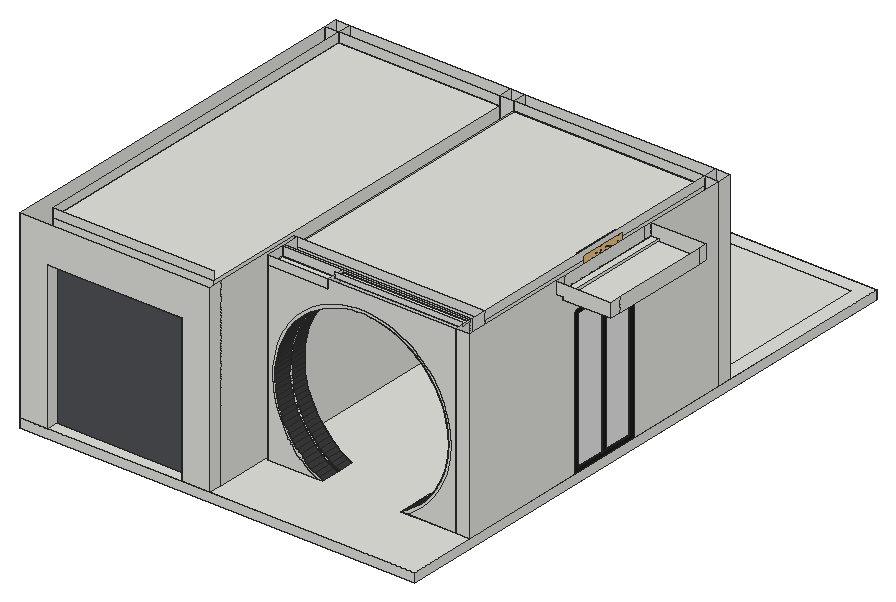
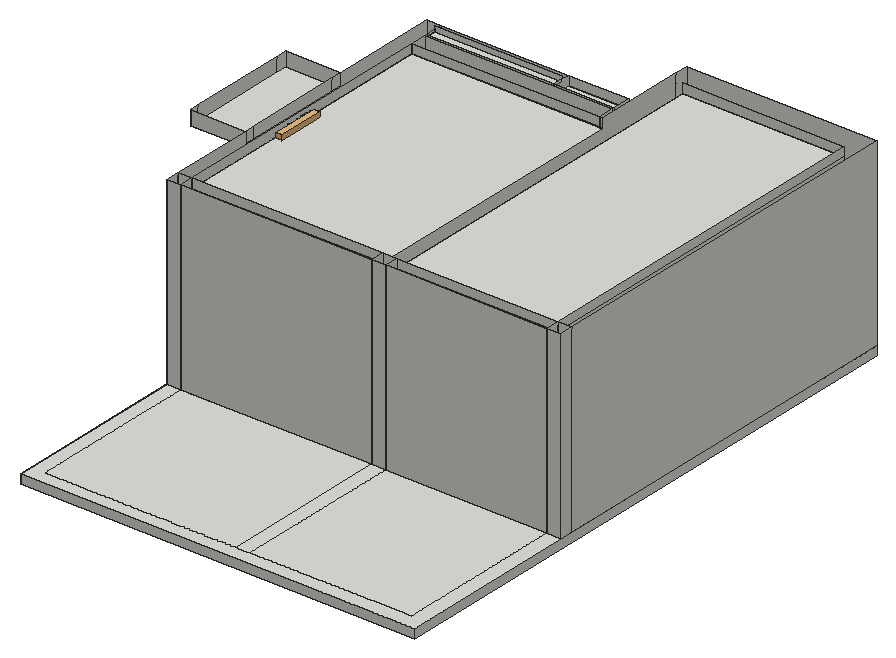
# SketchUp Ruby script. Lengths in inches.
U = 1.inch
M = Sketchup.active_model
def pt(a) = Geom::Point3d.new(a.map { |v| v * U })
def face(e, loops, mat)
  f = e.add_face(loops[0].map { |a| pt(a) })
  loops[1..].each { |l| e.add_face(l.map { |a| pt(a) }).erase! }
  f.material = f.back_material = mat if mat
  f
end
# faces: each face lists its corners as indices into pts; further lists are holes
def faces(e, pts, list, mat = nil) = list.each { |f| face(e, (f[0].is_a?(Array) ? f : [f]).map { |l| l.map { |i| pts[i] } }, mat) }
# xy, xz, yz: faces in a plane at the given z, y or x. An outline is a flat list of corners, or four numbers for a rectangle; further outlines are holes
def ring(l) = l.size == 4 ? [[l[0], l[1]], [l[2], l[1]], [l[2], l[3]], [l[0], l[3]]] : l.each_slice(2).to_a
def flat(e, list, mat, &to3) = list.each { |f| face(e, (f[0].is_a?(Array) ? f : [f]).map { |l| ring(l).map { |u, v| to3.(u, v) } }, mat) }
def xy(e, z, list, mat = nil) = flat(e, list, mat) { |x, y| [x, y, z] }
def xz(e, y, list, mat = nil) = flat(e, list, mat) { |x, z| [x, y, z] }
def yz(e, x, list, mat = nil) = flat(e, list, mat) { |y, z| [x, y, z] }
def lines(e, pts, list) = list.each { |a, b| e.add_line(pt(pts[a]), pt(pts[b])) }
# prism: a flat outline (further loops are holes) pulled along v
def prism(e, loops, v, mat = nil)
  f = face(e, loops, mat); d = Geom::Vector3d.new(v.map { |x| x * U })
  f.pushpull(f.normal.samedirection?(d) ? d.length : -d.length)
end
def box(e, o, s, mat = nil) = prism(e, [[o, [o[0] + s[0], o[1], o[2]], [o[0] + s[0], o[1] + s[1], o[2]], [o[0], o[1] + s[1], o[2]]]], [0, 0, s[2]], mat)
def at(x, y, z, deg = 0) = Geom::Transformation.translation(pt([x, y, z])) * Geom::Transformation.rotation(ORIGIN, Z_AXIS, deg.degrees)
def axes(o, x, y, z) = Geom::Transformation.new([*x, 0, *y, 0, *z, 0, *pt(o).to_a, 1])
def part(name) = M.definitions.add(name)
# library, detail: a bought-in or finely detailed component or shape, given as its bounding box
def library(name, o, s) = part(name).tap { |d| box(d.entities, o, s) }
def detail(e, o, s) = box(e.add_group.entities, o, s)
def put(e, d, t, mat = nil) = e.add_instance(d, t).tap { |i| i.material = mat if mat }
def group(e, t, mat = nil) = e.add_group.tap { |g| g.transformation = t; g.material = mat if mat }.entities
root = M.entities
M.materials.add("[Blinds Roman Hobbled Blue]").color = [81, 82, 87]
M.materials.add("[Color M07]").color = [58, 58, 58]
M.materials.add("[Color M08]").color = [30, 30, 30]
M.materials.add("[Mirror 02]").color = [229, 229, 229]
c1 = library("Curtains 004",[-15.59,-2.26,0],[31.18,4.52,116.91])
xy(root,-6,[[0,37.13,258,415.13]])
xy(root,0,[[0,37.13,18,37.13,18,44.38,106,44.38,106,37.13,124,37.13,124,286.13,115,286.13,115,52.07,9,52.07,9,286.13,0,286.13],[18,37.13,106,44.38],[[124,37.13,258,37.13,258,82.13,213,82.13,213,106.13,249,106.13,249,286.13,124,286.13],[126,82.13,162,106.13]],[9,52.07,115,286.13],[126,82.13,162,94.13],
  [213,82.13,249,94.13],[249,82.13,258,168.32],[126,94.13,162,95.7],[213,94.13,249,95.7],[126,95.7,162,106.13],
  [213,95.7,249,106.13],[249,216.32,258,286.13],[0,286.13,9,295.13],[9,286.13,115,295.13],[115,286.13,124,295.13],
  [124,286.13,249,295.13],[249,286.13,258,295.13],[0,295.13,9,295.13,9,406.13,249,406.13,249,295.13,258,295.13,258,415.13,0,415.13],[9,295.13,115,406.13],[115,295.13,124,406.13],
  [124,295.13,249,406.13]])
xy(root,0,[[254.4375,168.32,258,216.32]],"[Color M08]")
xy(root,2.75,[[256.5625,171.07,258,191.29],[256.5625,193.38,258,213.57]],"[Color M08]")
xy(root,93.25,[[256.5625,171.07,258,191.29],[256.5625,193.38,258,213.57]])
xy(root,96,[[18,37.13,106,44.38],[249,168.32,254.4375,216.32]])
xy(root,96,[[254.4375,168.32,258,216.32]],"[Color M08]")
xy(root,110.875,[[262.9375,152.76,294,230.88]])
xy(root,112.4375,[[258,152.76,262.9375,230.88]])
xy(root,114,[[9,52.07,115,286.13],[126,82.13,165.63,94.13],[124,106.13,249,286.13]])
xy(root,118.5,[[165.63,87.25,249,94.13]])
xz(root,37.13,[[0,-6,258,0],[0,0,18,0,18,96,106,96,106,0,124,0,124,120,0,120]])
xz(root,44.38,[[18,0,106,96]],"[Blinds Roman Hobbled Blue]")
xz(root,52.07,[[9,0,115,114],[9,114,115,120]])
xz(root,82.13,[[126,0,157.89,0,154.74,1.98,153.07,3.125,150.57,5.04,148.18,7.08,145.9,9.24,143.75,11.53,141.72,13.92,139.8125,16.42,138.05,19.02,136.43,21.71,134.95,24.49,133.62,27.33,132.45,30.25,131.4375,33.22,130.58,36.25,129.89,39.3125,129.36,42.41,129,45.53,128.8125,48.67,128.79,51.81,128.93,54.95,129.24,58.07,129.72,61.18,130.36,64.25,131.17,67.29,132.14,70.28,133.27,73.21,134.55,76.08,135.98,78.875,137.5625,81.59,139.29,84.22,141.15,86.75,143.14,89.18,145.27,91.49,147.51,93.69,149.87,95.77,152.33,97.72,154.9,99.53,157.56,101.21,160.3,102.74,163.12,104.12,166.01,105.34,168.97,106.41,171.98,107.33,175.03,108.08,178.11,108.66,181.23,109.08,184.36,109.33,187.5,109.42,190.64,109.33,193.77,109.08,196.89,108.66,199.97,108.08,203.02,107.33,206.03,106.41,208.99,105.34,211.88,104.12,214.7,102.74,217.44,101.21,220.1,99.53,222.67,97.72,225.13,95.77,227.49,93.69,229.73,91.49,231.86,89.18,233.85,86.75,235.71,84.22,237.4375,81.59,239.02,78.875,240.45,76.08,241.73,73.21,242.86,70.28,243.83,67.29,244.64,64.25,245.28,61.18,245.76,58.07,246.07,54.95,246.21,51.81,246.1875,48.67,246,45.53,245.64,42.41,245.11,39.3125,244.42,36.25,243.5625,33.22,242.55,30.25,241.38,27.33,240.05,24.49,238.57,21.71,236.95,19.02,235.1875,16.42,233.28,13.92,231.25,11.53,229.1,9.24,226.82,7.08,224.43,5.04,221.93,3.125,220.26,1.98,217.36,0,249,0,249,120,165.63,120,165.63,114,126,114],[157.89,0,162,0,159.33,1.4375,156.73,3.01,154.23,4.73,151.8125,6.57,149.51,8.55,147.31,10.64,145.22,12.84,143.26,15.16,141.42,17.58,139.71,20.09,138.15,22.6875,136.72,25.37,135.4375,28.12,134.3,30.9375,133.32,33.8125,132.5,36.73,131.83,39.69,131.32,42.6875,130.97,45.7,130.79,48.73,130.77,51.77,130.9,54.8,131.21,57.82,131.67,60.83,132.29,63.8,133.07,66.73,134,69.62,135.09,72.45,136.33,75.23,137.72,77.93,139.25,80.55,140.91,83.09,142.71,85.53,144.64,87.88,146.6875,90.12,148.86,92.25,151.13,94.25,153.52,96.14,155.99,97.89,158.5625,99.51,161.22,100.98,163.94,102.32,166.74,103.5,169.59,104.54,172.5,105.42,175.45,106.14,178.43,106.71,181.4375,107.11,184.47,107.36,187.5,107.4375,190.53,107.36,193.5625,107.11,196.57,106.71,199.55,106.14,202.5,105.42,205.41,104.54,208.26,103.5,211.06,102.32,213.78,100.98,216.4375,99.51,219.01,97.89,221.48,96.14,223.87,94.25,226.14,92.25,228.3125,90.12,230.36,87.88,232.29,85.53,234.09,83.09,235.75,80.55,237.28,77.93,238.67,75.23,239.91,72.45,241,69.62,241.93,66.73,242.71,63.8,243.33,60.83,243.79,57.82,244.1,54.8,244.23,51.77,244.21,48.73,244.03,45.7,243.68,42.6875,243.17,39.69,242.5,36.73,241.68,33.8125,240.7,30.9375,239.5625,28.12,238.28,25.37,236.85,22.6875,235.29,20.09,233.58,17.58,231.74,15.16,229.78,12.84,227.69,10.64,225.49,8.55,223.1875,6.57,220.77,4.73,218.27,3.01,215.67,1.4375,213,0,217.36,0,220.26,1.98,221.93,3.125,224.43,5.04,226.82,7.08,229.1,9.24,231.25,11.53,233.28,13.92,235.1875,16.42,236.95,19.02,238.57,21.71,240.05,24.49,241.38,27.33,242.55,30.25,243.5625,33.22,244.42,36.25,245.11,39.3125,245.64,42.41,246,45.53,246.1875,48.67,246.21,51.81,246.07,54.95,245.76,58.07,245.28,61.18,244.64,64.25,243.83,67.29,242.86,70.28,241.73,73.21,240.45,76.08,239.02,78.875,237.4375,81.59,235.71,84.22,233.85,86.75,231.86,89.18,229.73,91.49,227.49,93.69,225.13,95.77,222.67,97.72,220.1,99.53,217.44,101.21,214.7,102.74,211.88,104.12,208.99,105.34,206.03,106.41,203.02,107.33,199.97,108.08,196.89,108.66,193.77,109.08,190.64,109.33,187.5,109.42,184.36,109.33,181.23,109.08,178.11,108.66,175.03,108.08,171.98,107.33,168.97,106.41,166.01,105.34,163.12,104.12,160.3,102.74,157.56,101.21,154.9,99.53,152.33,97.72,149.87,95.77,147.51,93.69,145.27,91.49,143.14,89.18,141.15,86.75,139.29,84.22,137.5625,81.59,135.98,78.875,134.55,76.08,133.27,73.21,132.14,70.28,131.17,67.29,130.36,64.25,129.72,61.18,129.24,58.07,128.93,54.95,128.79,51.81,128.8125,48.67,129,45.53,129.36,42.41,129.89,39.3125,130.58,36.25,131.4375,33.22,132.45,30.25,133.62,27.33,134.95,24.49,136.43,21.71,138.05,19.02,139.8125,16.42,141.72,13.92,143.75,11.53,145.9,9.24,148.18,7.08,150.57,5.04,153.07,3.125,154.74,1.98],[249,0,258,120],[126,114,165.63,120]])
xz(root,87.25,[[165.63,118.5,249,122]])
xz(root,94.13,[[126,0,126,114,165.63,114,165.63,118.5,249,118.5,249,0,213,0,215.67,1.4375,218.27,3.01,220.77,4.73,223.1875,6.57,225.49,8.55,227.69,10.64,229.78,12.84,231.74,15.16,233.58,17.58,235.29,20.09,236.85,22.6875,238.28,25.37,239.5625,28.12,240.7,30.9375,241.68,33.8125,242.5,36.73,243.17,39.69,243.68,42.6875,244.03,45.7,244.21,48.73,244.23,51.77,244.1,54.8,243.79,57.82,243.33,60.83,242.71,63.8,241.93,66.73,241,69.62,239.91,72.45,238.67,75.23,237.28,77.93,235.75,80.55,234.09,83.09,232.29,85.53,230.36,87.88,228.3125,90.12,226.14,92.25,223.87,94.25,221.48,96.14,219.01,97.89,216.4375,99.51,213.78,100.98,211.06,102.32,208.26,103.5,205.41,104.54,202.5,105.42,199.55,106.14,196.57,106.71,193.5625,107.11,190.53,107.36,187.5,107.4375,184.47,107.36,181.4375,107.11,178.43,106.71,175.45,106.14,172.5,105.42,169.59,104.54,166.74,103.5,163.94,102.32,161.22,100.98,158.5625,99.51,155.99,97.89,153.52,96.14,151.13,94.25,148.86,92.25,146.6875,90.12,144.64,87.88,142.71,85.53,140.91,83.09,139.25,80.55,137.72,77.93,136.33,75.23,135.09,72.45,134,69.62,133.07,66.73,132.29,63.8,131.67,60.83,131.21,57.82,130.9,54.8,130.77,51.77,130.79,48.73,130.97,45.7,131.32,42.6875,131.83,39.69,132.5,36.73,133.32,33.8125,134.3,30.9375,135.4375,28.12,136.72,25.37,138.15,22.6875,139.71,20.09,141.42,17.58,143.26,15.16,145.22,12.84,147.31,10.64,149.51,8.55,151.8125,6.57,154.23,4.73,156.73,3.01,159.33,1.4375,162,0],[126,114,165.63,120],[165.63,118.5,249,120]])
xz(root,95.7,[[126,0,126,120,249,120,249,0,213,0,215.67,1.4375,218.27,3.01,220.77,4.73,223.1875,6.57,225.49,8.55,227.69,10.64,229.78,12.84,231.74,15.16,233.58,17.58,235.29,20.09,236.85,22.6875,238.28,25.37,239.5625,28.12,240.7,30.9375,241.68,33.8125,242.5,36.73,243.17,39.69,243.68,42.6875,244.03,45.7,244.21,48.73,244.23,51.77,244.1,54.8,243.79,57.82,243.33,60.83,242.71,63.8,241.93,66.73,241,69.62,239.91,72.45,238.67,75.23,237.28,77.93,235.75,80.55,234.09,83.09,232.29,85.53,230.36,87.88,228.3125,90.12,226.14,92.25,223.87,94.25,221.48,96.14,219.01,97.89,216.4375,99.51,213.78,100.98,211.06,102.32,208.26,103.5,205.41,104.54,202.5,105.42,199.55,106.14,196.57,106.71,193.5625,107.11,190.53,107.36,187.5,107.4375,184.47,107.36,181.4375,107.11,178.43,106.71,175.45,106.14,172.5,105.42,169.59,104.54,166.74,103.5,163.94,102.32,161.22,100.98,158.5625,99.51,155.99,97.89,153.52,96.14,151.13,94.25,148.86,92.25,146.6875,90.12,144.64,87.88,142.71,85.53,140.91,83.09,139.25,80.55,137.72,77.93,136.33,75.23,135.09,72.45,134,69.62,133.07,66.73,132.29,63.8,131.67,60.83,131.21,57.82,130.9,54.8,130.77,51.77,130.79,48.73,130.97,45.7,131.32,42.6875,131.83,39.69,132.5,36.73,133.32,33.8125,134.3,30.9375,135.4375,28.12,136.72,25.37,138.15,22.6875,139.71,20.09,141.42,17.58,143.26,15.16,145.22,12.84,147.31,10.64,149.51,8.55,151.8125,6.57,154.23,4.73,156.73,3.01,159.33,1.4375,162,0]])
xz(root,106.13,[[126,0,126,114,249,114,249,0,213,0,215.67,1.4375,218.27,3.01,220.77,4.73,223.1875,6.57,225.49,8.55,227.69,10.64,229.78,12.84,231.74,15.16,233.58,17.58,235.29,20.09,236.85,22.6875,238.28,25.37,239.5625,28.12,240.7,30.9375,241.68,33.8125,242.5,36.73,243.17,39.69,243.68,42.6875,244.03,45.7,244.21,48.73,244.23,51.77,244.1,54.8,243.79,57.82,243.33,60.83,242.71,63.8,241.93,66.73,241,69.62,239.91,72.45,238.67,75.23,237.28,77.93,235.75,80.55,234.09,83.09,232.29,85.53,230.36,87.88,228.3125,90.12,226.14,92.25,223.87,94.25,221.48,96.14,219.01,97.89,216.4375,99.51,213.78,100.98,211.06,102.32,208.26,103.5,205.41,104.54,202.5,105.42,199.55,106.14,196.57,106.71,193.5625,107.11,190.53,107.36,187.5,107.4375,184.47,107.36,181.4375,107.11,178.43,106.71,175.45,106.14,172.5,105.42,169.59,104.54,166.74,103.5,163.94,102.32,161.22,100.98,158.5625,99.51,155.99,97.89,153.52,96.14,151.13,94.25,148.86,92.25,146.6875,90.12,144.64,87.88,142.71,85.53,140.91,83.09,139.25,80.55,137.72,77.93,136.33,75.23,135.09,72.45,134,69.62,133.07,66.73,132.29,63.8,131.67,60.83,131.21,57.82,130.9,54.8,130.77,51.77,130.79,48.73,130.97,45.7,131.32,42.6875,131.83,39.69,132.5,36.73,133.32,33.8125,134.3,30.9375,135.4375,28.12,136.72,25.37,138.15,22.6875,139.71,20.09,141.42,17.58,143.26,15.16,145.22,12.84,147.31,10.64,149.51,8.55,151.8125,6.57,154.23,4.73,156.73,3.01,159.33,1.4375,162,0],[124,114,126,120],[126,114,249,120]])
xz(root,152.76,[[262.9375,110.875,294,110.875,294,120,258,120,258,112.4375,262.9375,112.4375]])
xz(root,168.32,[[249,0,254.4375,96]])
xz(root,168.32,[[254.4375,0,258,96]],"[Color M08]")
xz(root,171.07,[[256.5625,2.75,258,93.25]],"[Color M08]")
xz(root,191.29,[[256.5625,2.75,258,93.25]],"[Color M08]")
xz(root,193.38,[[256.5625,2.75,258,93.25]],"[Color M08]")
xz(root,213.57,[[256.5625,2.75,258,93.25]],"[Color M08]")
xz(root,216.32,[[249,0,254.4375,96]])
xz(root,216.32,[[254.4375,0,258,96]],"[Color M08]")
xz(root,230.88,[[262.9375,110.875,262.9375,112.4375,258,112.4375,258,120,294,120,294,110.875]])
xz(root,286.13,[[0,0,9,120],[9,0,115,114],[115,0,124,120],[124,0,249,114],[249,0,258,120],
  [9,114,115,120],[124,114,249,120]])
xz(root,295.13,[[0,0,9,120],[9,0,115,120],[115,0,124,120],[124,0,249,120],[249,0,258,120]])
xz(root,415.13,[[0,-6,258,0]])
yz(root,0,[[37.13,-6,415.13,0],[37.13,0,286.13,120],[286.13,0,295.13,120]])
yz(root,9,[[52.07,0,286.13,114],[286.13,0,295.13,120],[52.07,114,286.13,120]])
yz(root,18,[[37.13,0,44.38,96]])
yz(root,106,[[37.13,0,44.38,96]])
yz(root,115,[[52.07,0,286.13,114],[286.13,0,295.13,120]])
yz(root,124,[[37.13,0,46.13,120],[46.13,0,286.13,0,286.13,114,106.13,114,106.13,120,46.13,120],[286.13,0,295.13,120]])
yz(root,126,[[82.13,0,94.13,114],[94.13,0,95.7,120],[95.7,0,106.13,120],[82.13,114,94.13,120]])
yz(root,165.63,[[82.13,114,94.13,114,94.13,118.5,87.25,118.5,87.25,120,82.13,120],[87.25,118.5,94.13,120]])
yz(root,249,[[82.13,0,94.13,0,94.13,118.5,87.25,118.5,87.25,120,82.13,120],[94.13,0,95.7,120],[95.7,0,106.13,120],[106.13,0,106.13,114,286.13,114,286.13,0,216.32,0,216.32,96,168.32,96,168.32,0],[286.13,0,295.13,120],
  [106.13,114,286.13,120],[87.25,118.5,94.13,120]])
yz(root,254.4375,[[168.32,0,216.32,96]],"[Mirror 02]")
yz(root,256.5625,[[171.07,2.75,191.29,93.25],[193.38,2.75,213.57,93.25]],"[Mirror 02]")
yz(root,258,[[37.13,-6,415.13,0],[82.13,0,168.32,0,168.32,96,216.32,96,216.32,0,286.13,0,286.13,120,230.88,120,230.88,112.4375,152.76,112.4375,152.76,120,82.13,120],[286.13,0,295.13,120],[152.76,112.4375,160.01,120],[160.01,112.4375,224.82,120],
  [224.82,112.4375,230.88,120]])
yz(root,258,[[[168.32,0,216.32,96],[171.07,2.75,213.57,93.25]],[191.29,2.75,193.38,93.25]],"[Color M08]")
yz(root,262.9375,[[152.76,110.875,230.88,112.4375]])
yz(root,294,[[152.76,110.875,160.01,120],[160.01,110.875,224.82,120],[224.82,110.875,230.88,120]])
p = [[162,82.13,0],[162,94.13,0],[159.33,94.13,1.4375],[159.33,82.13,1.4375],[215.67,82.13,1.4375],[215.67,94.13,1.4375],
  [213,94.13,0],[213,82.13,0],[162,95.7,0],[159.33,95.7,1.4375],[215.67,95.7,1.4375],[213,95.7,0],
  [159.33,106.13,1.4375],[162,106.13,0],[213,106.13,0],[215.67,106.13,1.4375],[156.73,94.13,3.01],[156.73,82.13,3.01],
  [218.27,82.13,3.01],[218.27,94.13,3.01],[156.73,95.7,3.01],[218.27,95.7,3.01],[156.73,106.13,3.01],[218.27,106.13,3.01],
  [154.23,94.13,4.73],[154.23,82.13,4.73],[220.77,82.13,4.73],[220.77,94.13,4.73],[154.23,95.7,4.73],[220.77,95.7,4.73],
  [154.23,106.13,4.73],[220.77,106.13,4.73],[151.8125,94.13,6.57],[151.8125,82.13,6.57],[223.1875,82.13,6.57],[223.1875,94.13,6.57],
  [151.8125,95.7,6.57],[223.1875,95.7,6.57],[151.8125,106.13,6.57],[223.1875,106.13,6.57],[149.51,94.13,8.55],[149.51,82.13,8.55],
  [225.49,82.13,8.55],[225.49,94.13,8.55],[149.51,95.7,8.55],[225.49,95.7,8.55],[149.51,106.13,8.55],[225.49,106.13,8.55],
  [147.31,94.13,10.64],[147.31,82.13,10.64],[227.69,82.13,10.64],[227.69,94.13,10.64],[147.31,95.7,10.64],[227.69,95.7,10.64],
  [147.31,106.13,10.64],[227.69,106.13,10.64],[145.22,94.13,12.84],[145.22,82.13,12.84],[229.78,82.13,12.84],[229.78,94.13,12.84],
  [145.22,95.7,12.84],[229.78,95.7,12.84],[145.22,106.13,12.84],[229.78,106.13,12.84],[143.26,94.13,15.16],[143.26,82.13,15.16],
  [231.74,82.13,15.16],[231.74,94.13,15.16],[143.26,95.7,15.16],[231.74,95.7,15.16],[143.26,106.13,15.16],[231.74,106.13,15.16],
  [141.42,94.13,17.58],[141.42,82.13,17.58],[233.58,82.13,17.58],[233.58,94.13,17.58],[141.42,95.7,17.58],[233.58,95.7,17.58],
  [141.42,106.13,17.58],[233.58,106.13,17.58],[139.71,94.13,20.09],[139.71,82.13,20.09],[235.29,82.13,20.09],[235.29,94.13,20.09],
  [139.71,95.7,20.09],[235.29,95.7,20.09],[139.71,106.13,20.09],[235.29,106.13,20.09],[138.15,94.13,22.6875],[138.15,82.13,22.6875],
  [236.85,82.13,22.6875],[236.85,94.13,22.6875],[138.15,95.7,22.6875],[236.85,95.7,22.6875],[138.15,106.13,22.6875],[236.85,106.13,22.6875],
  [136.72,94.13,25.37],[136.72,82.13,25.37],[238.28,82.13,25.37],[238.28,94.13,25.37],[136.72,95.7,25.37],[238.28,95.7,25.37],
  [136.72,106.13,25.37],[238.28,106.13,25.37],[135.4375,94.13,28.12],[135.4375,82.13,28.12],[239.5625,82.13,28.12],[239.5625,94.13,28.12],
  [135.4375,95.7,28.12],[239.5625,95.7,28.12],[135.4375,106.13,28.12],[239.5625,106.13,28.12],[134.3,94.13,30.9375],[134.3,82.13,30.9375],
  [240.7,82.13,30.9375],[240.7,94.13,30.9375],[134.3,95.7,30.9375],[240.7,95.7,30.9375],[134.3,106.13,30.9375],[240.7,106.13,30.9375],
  [133.32,94.13,33.8125],[133.32,82.13,33.8125],[241.68,82.13,33.8125],[241.68,94.13,33.8125],[133.32,95.7,33.8125],[241.68,95.7,33.8125],
  [133.32,106.13,33.8125],[241.68,106.13,33.8125],[132.5,94.13,36.73],[132.5,82.13,36.73],[242.5,82.13,36.73],[242.5,94.13,36.73],
  [132.5,95.7,36.73],[242.5,95.7,36.73],[132.5,106.13,36.73],[242.5,106.13,36.73],[131.83,94.13,39.69],[131.83,82.13,39.69],
  [243.17,82.13,39.69],[243.17,94.13,39.69],[131.83,95.7,39.69],[243.17,95.7,39.69],[131.83,106.13,39.69],[243.17,106.13,39.69],
  [131.32,94.13,42.6875],[131.32,82.13,42.6875],[243.68,82.13,42.6875],[243.68,94.13,42.6875],[131.32,95.7,42.6875],[243.68,95.7,42.6875],
  [131.32,106.13,42.6875],[243.68,106.13,42.6875],[130.97,94.13,45.7],[130.97,82.13,45.7],[244.03,82.13,45.7],[244.03,94.13,45.7],
  [130.97,95.7,45.7],[244.03,95.7,45.7],[130.97,106.13,45.7],[244.03,106.13,45.7],[130.79,94.13,48.73],[130.79,82.13,48.73],
  [244.21,82.13,48.73],[244.21,94.13,48.73],[130.79,95.7,48.73],[244.21,95.7,48.73],[130.79,106.13,48.73],[244.21,106.13,48.73],
  [130.77,94.13,51.77],[130.77,82.13,51.77],[244.23,82.13,51.77],[244.23,94.13,51.77],[130.77,95.7,51.77],[244.23,95.7,51.77],
  [130.77,106.13,51.77],[244.23,106.13,51.77],[130.9,94.13,54.8],[130.9,82.13,54.8],[244.1,82.13,54.8],[244.1,94.13,54.8],
  [130.9,95.7,54.8],[244.1,95.7,54.8],[130.9,106.13,54.8],[244.1,106.13,54.8],[131.21,94.13,57.82],[131.21,82.13,57.82],
  [243.79,82.13,57.82],[243.79,94.13,57.82],[131.21,95.7,57.82],[243.79,95.7,57.82],[131.21,106.13,57.82],[243.79,106.13,57.82],
  [131.67,94.13,60.83],[131.67,82.13,60.83],[243.33,82.13,60.83],[243.33,94.13,60.83],[131.67,95.7,60.83],[243.33,95.7,60.83],
  [131.67,106.13,60.83],[243.33,106.13,60.83],[132.29,94.13,63.8],[132.29,82.13,63.8],[242.71,82.13,63.8],[242.71,94.13,63.8],
  [132.29,95.7,63.8],[242.71,95.7,63.8],[132.29,106.13,63.8],[242.71,106.13,63.8],[133.07,94.13,66.73],[133.07,82.13,66.73],
  [241.93,82.13,66.73],[241.93,94.13,66.73],[133.07,95.7,66.73],[241.93,95.7,66.73],[133.07,106.13,66.73],[241.93,106.13,66.73],
  [134,94.13,69.62],[134,82.13,69.62],[241,82.13,69.62],[241,94.13,69.62],[134,95.7,69.62],[241,95.7,69.62],
  [134,106.13,69.62],[241,106.13,69.62],[135.09,94.13,72.45],[135.09,82.13,72.45],[239.91,82.13,72.45],[239.91,94.13,72.45],
  [135.09,95.7,72.45],[239.91,95.7,72.45],[135.09,106.13,72.45],[239.91,106.13,72.45],[136.33,94.13,75.23],[136.33,82.13,75.23],
  [238.67,82.13,75.23],[238.67,94.13,75.23],[136.33,95.7,75.23],[238.67,95.7,75.23],[136.33,106.13,75.23],[238.67,106.13,75.23],
  [137.72,94.13,77.93],[137.72,82.13,77.93],[237.28,82.13,77.93],[237.28,94.13,77.93],[137.72,95.7,77.93],[237.28,95.7,77.93],
  [137.72,106.13,77.93],[237.28,106.13,77.93],[139.25,94.13,80.55],[139.25,82.13,80.55],[235.75,82.13,80.55],[235.75,94.13,80.55],
  [139.25,95.7,80.55],[235.75,95.7,80.55],[139.25,106.13,80.55],[235.75,106.13,80.55],[140.91,94.13,83.09],[140.91,82.13,83.09],
  [234.09,82.13,83.09],[234.09,94.13,83.09],[140.91,95.7,83.09],[234.09,95.7,83.09],[140.91,106.13,83.09],[234.09,106.13,83.09],
  [142.71,94.13,85.53],[142.71,82.13,85.53],[232.29,82.13,85.53],[232.29,94.13,85.53],[142.71,95.7,85.53],[232.29,95.7,85.53],
  [142.71,106.13,85.53],[232.29,106.13,85.53],[144.64,94.13,87.88],[144.64,82.13,87.88],[230.36,82.13,87.88],[230.36,94.13,87.88],
  [144.64,95.7,87.88],[230.36,95.7,87.88],[144.64,106.13,87.88],[230.36,106.13,87.88],[146.6875,94.13,90.12],[146.6875,82.13,90.12],
  [228.3125,82.13,90.12],[228.3125,94.13,90.12],[146.6875,95.7,90.12],[228.3125,95.7,90.12],[146.6875,106.13,90.12],[228.3125,106.13,90.12],
  [148.86,94.13,92.25],[148.86,82.13,92.25],[226.14,82.13,92.25],[226.14,94.13,92.25],[148.86,95.7,92.25],[226.14,95.7,92.25],
  [148.86,106.13,92.25],[226.14,106.13,92.25],[151.13,94.13,94.25],[151.13,82.13,94.25],[223.87,82.13,94.25],[223.87,94.13,94.25],
  [151.13,95.7,94.25],[223.87,95.7,94.25],[151.13,106.13,94.25],[223.87,106.13,94.25],[153.52,94.13,96.14],[153.52,82.13,96.14],
  [221.48,82.13,96.14],[221.48,94.13,96.14],[153.52,95.7,96.14],[221.48,95.7,96.14],[153.52,106.13,96.14],[221.48,106.13,96.14],
  [155.99,94.13,97.89],[155.99,82.13,97.89],[219.01,82.13,97.89],[219.01,94.13,97.89],[155.99,95.7,97.89],[219.01,95.7,97.89],
  [155.99,106.13,97.89],[219.01,106.13,97.89],[158.5625,94.13,99.51],[158.5625,82.13,99.51],[216.4375,82.13,99.51],[216.4375,94.13,99.51],
  [158.5625,95.7,99.51],[216.4375,95.7,99.51],[158.5625,106.13,99.51],[216.4375,106.13,99.51],[161.22,94.13,100.98],[161.22,82.13,100.98],
  [213.78,82.13,100.98],[213.78,94.13,100.98],[161.22,95.7,100.98],[213.78,95.7,100.98],[161.22,106.13,100.98],[213.78,106.13,100.98],
  [163.94,94.13,102.32],[163.94,82.13,102.32],[211.06,82.13,102.32],[211.06,94.13,102.32],[163.94,95.7,102.32],[211.06,95.7,102.32],
  [163.94,106.13,102.32],[211.06,106.13,102.32],[166.74,94.13,103.5],[166.74,82.13,103.5],[208.26,82.13,103.5],[208.26,94.13,103.5],
  [166.74,95.7,103.5],[208.26,95.7,103.5],[166.74,106.13,103.5],[208.26,106.13,103.5],[169.59,94.13,104.54],[169.59,82.13,104.54],
  [205.41,82.13,104.54],[205.41,94.13,104.54],[169.59,95.7,104.54],[205.41,95.7,104.54],[169.59,106.13,104.54],[205.41,106.13,104.54],
  [172.5,94.13,105.42],[172.5,82.13,105.42],[202.5,82.13,105.42],[202.5,94.13,105.42],[172.5,95.7,105.42],[202.5,95.7,105.42],
  [172.5,106.13,105.42],[202.5,106.13,105.42],[175.45,94.13,106.14],[175.45,82.13,106.14],[199.55,82.13,106.14],[199.55,94.13,106.14],
  [175.45,95.7,106.14],[199.55,95.7,106.14],[175.45,106.13,106.14],[199.55,106.13,106.14],[178.43,94.13,106.71],[178.43,82.13,106.71],
  [196.57,82.13,106.71],[196.57,94.13,106.71],[178.43,95.7,106.71],[196.57,95.7,106.71],[178.43,106.13,106.71],[196.57,106.13,106.71],
  [181.4375,94.13,107.11],[181.4375,82.13,107.11],[193.5625,82.13,107.11],[193.5625,94.13,107.11],[181.4375,95.7,107.11],[193.5625,95.7,107.11],
  [181.4375,106.13,107.11],[193.5625,106.13,107.11],[184.47,94.13,107.36],[184.47,82.13,107.36],[190.53,82.13,107.36],[190.53,94.13,107.36],
  [184.47,95.7,107.36],[190.53,95.7,107.36],[184.47,106.13,107.36],[190.53,106.13,107.36],[187.5,94.13,107.4375],[187.5,82.13,107.4375],
  [187.5,95.7,107.4375],[187.5,106.13,107.4375]]
faces(root,p,[[0,1,2,3],[4,5,6,7],[12,9,8,13],[14,11,10,15],[3,2,16,17],[18,19,5,4],[22,20,9,12],[15,10,21,23],
  [17,16,24,25],[26,27,19,18],[30,28,20,22],[23,21,29,31],[25,24,32,33],[34,35,27,26],[38,36,28,30],[31,29,37,39],
  [33,32,40,41],[42,43,35,34],[46,44,36,38],[39,37,45,47],[41,40,48,49],[50,51,43,42],[54,52,44,46],[47,45,53,55],
  [49,48,56,57],[58,59,51,50],[62,60,52,54],[55,53,61,63],[57,56,64,65],[66,67,59,58],[70,68,60,62],[63,61,69,71],
  [65,64,72,73],[74,75,67,66],[78,76,68,70],[71,69,77,79],[73,72,80,81],[82,83,75,74],[86,84,76,78],[79,77,85,87],
  [81,80,88,89],[90,91,83,82],[94,92,84,86],[87,85,93,95],[89,88,96,97],[98,99,91,90],[102,100,92,94],[95,93,101,103],
  [97,96,104,105],[106,107,99,98],[110,108,100,102],[103,101,109,111],[105,104,112,113],[114,115,107,106],[118,116,108,110],[111,109,117,119],
  [113,112,120,121],[122,123,115,114],[126,124,116,118],[119,117,125,127],[121,120,128,129],[130,131,123,122],[134,132,124,126],[127,125,133,135],
  [129,128,136,137],[138,139,131,130],[142,140,132,134],[135,133,141,143],[137,136,144,145],[146,147,139,138],[150,148,140,142],[143,141,149,151],
  [145,144,152,153],[154,155,147,146],[158,156,148,150],[151,149,157,159],[153,152,160,161],[162,163,155,154],[166,164,156,158],[159,157,165,167],
  [161,160,168,169],[170,171,163,162],[174,172,164,166],[167,165,173,175],[169,168,176,177],[178,179,171,170],[182,180,172,174],[175,173,181,183],
  [177,176,184,185],[186,187,179,178],[190,188,180,182],[183,181,189,191],[185,184,192,193],[194,195,187,186],[198,196,188,190],[191,189,197,199],
  [193,192,200,201],[202,203,195,194],[206,204,196,198],[199,197,205,207],[201,200,208,209],[210,211,203,202],[214,212,204,206],[207,205,213,215],
  [209,208,216,217],[218,219,211,210],[222,220,212,214],[215,213,221,223],[217,216,224,225],[226,227,219,218],[230,228,220,222],[223,221,229,231],
  [225,224,232,233],[234,235,227,226],[238,236,228,230],[231,229,237,239],[233,232,240,241],[242,243,235,234],[246,244,236,238],[239,237,245,247],
  [241,240,248,249],[250,251,243,242],[254,252,244,246],[247,245,253,255],[249,248,256,257],[258,259,251,250],[262,260,252,254],[255,253,261,263],
  [257,256,264,265],[266,267,259,258],[270,268,260,262],[263,261,269,271],[265,264,272,273],[274,275,267,266],[278,276,268,270],[271,269,277,279],
  [273,272,280,281],[282,283,275,274],[286,284,276,278],[279,277,285,287],[281,280,288,289],[290,291,283,282],[294,292,284,286],[287,285,293,295],
  [289,288,296,297],[298,299,291,290],[302,300,292,294],[295,293,301,303],[297,296,304,305],[306,307,299,298],[310,308,300,302],[303,301,309,311],
  [305,304,312,313],[314,315,307,306],[318,316,308,310],[311,309,317,319],[313,312,320,321],[322,323,315,314],[326,324,316,318],[319,317,325,327],
  [321,320,328,329],[330,331,323,322],[334,332,324,326],[327,325,333,335],[329,328,336,337],[338,339,331,330],[342,340,332,334],[335,333,341,343],
  [337,336,344,345],[346,347,339,338],[350,348,340,342],[343,341,349,351],[345,344,352,353],[354,355,347,346],[358,356,348,350],[351,349,357,359],
  [353,352,360,361],[362,363,355,354],[366,364,356,358],[359,357,365,367],[361,360,368,369],[370,371,363,362],[374,372,364,366],[367,365,373,375],
  [369,368,376,377],[378,379,371,370],[382,380,372,374],[375,373,381,383],[377,376,384,385],[386,387,379,378],[390,388,380,382],[383,381,389,391],
  [385,384,392,393],[394,395,387,386],[398,396,388,390],[391,389,397,399],[393,392,400,401],[401,400,395,394],[403,402,396,398],[399,397,402,403]],"[Color M07]")
faces(root,p,[[1,8,9,2],[5,10,11,6],[2,9,20,16],[19,21,10,5],[16,20,28,24],[27,29,21,19],[24,28,36,32],[35,37,29,27],
  [32,36,44,40],[43,45,37,35],[40,44,52,48],[51,53,45,43],[48,52,60,56],[59,61,53,51],[56,60,68,64],[67,69,61,59],
  [64,68,76,72],[75,77,69,67],[72,76,84,80],[83,85,77,75],[80,84,92,88],[91,93,85,83],[88,92,100,96],[99,101,93,91],
  [96,100,108,104],[107,109,101,99],[104,108,116,112],[115,117,109,107],[112,116,124,120],[123,125,117,115],[120,124,132,128],[131,133,125,123],
  [128,132,140,136],[139,141,133,131],[136,140,148,144],[147,149,141,139],[144,148,156,152],[155,157,149,147],[152,156,164,160],[163,165,157,155],
  [160,164,172,168],[171,173,165,163],[168,172,180,176],[179,181,173,171],[176,180,188,184],[187,189,181,179],[184,188,196,192],[195,197,189,187],
  [192,196,204,200],[203,205,197,195],[200,204,212,208],[211,213,205,203],[208,212,220,216],[219,221,213,211],[216,220,228,224],[227,229,221,219],
  [224,228,236,232],[235,237,229,227],[232,236,244,240],[243,245,237,235],[240,244,252,248],[251,253,245,243],[248,252,260,256],[259,261,253,251],
  [256,260,268,264],[267,269,261,259],[264,268,276,272],[275,277,269,267],[272,276,284,280],[283,285,277,275],[280,284,292,288],[291,293,285,283],
  [288,292,300,296],[299,301,293,291],[296,300,308,304],[307,309,301,299],[304,308,316,312],[315,317,309,307],[312,316,324,320],[323,325,317,315],
  [320,324,332,328],[331,333,325,323],[328,332,340,336],[339,341,333,331],[336,340,348,344],[347,349,341,339],[344,348,356,352],[355,357,349,347],
  [352,356,364,360],[363,365,357,355],[360,364,372,368],[371,373,365,363],[368,372,380,376],[379,381,373,371],[376,380,388,384],[387,389,381,379],
  [384,388,396,392],[395,397,389,387],[392,396,402,400],[400,402,397,395]])
put(root,c1,at(246.74,202.23,0,90))
